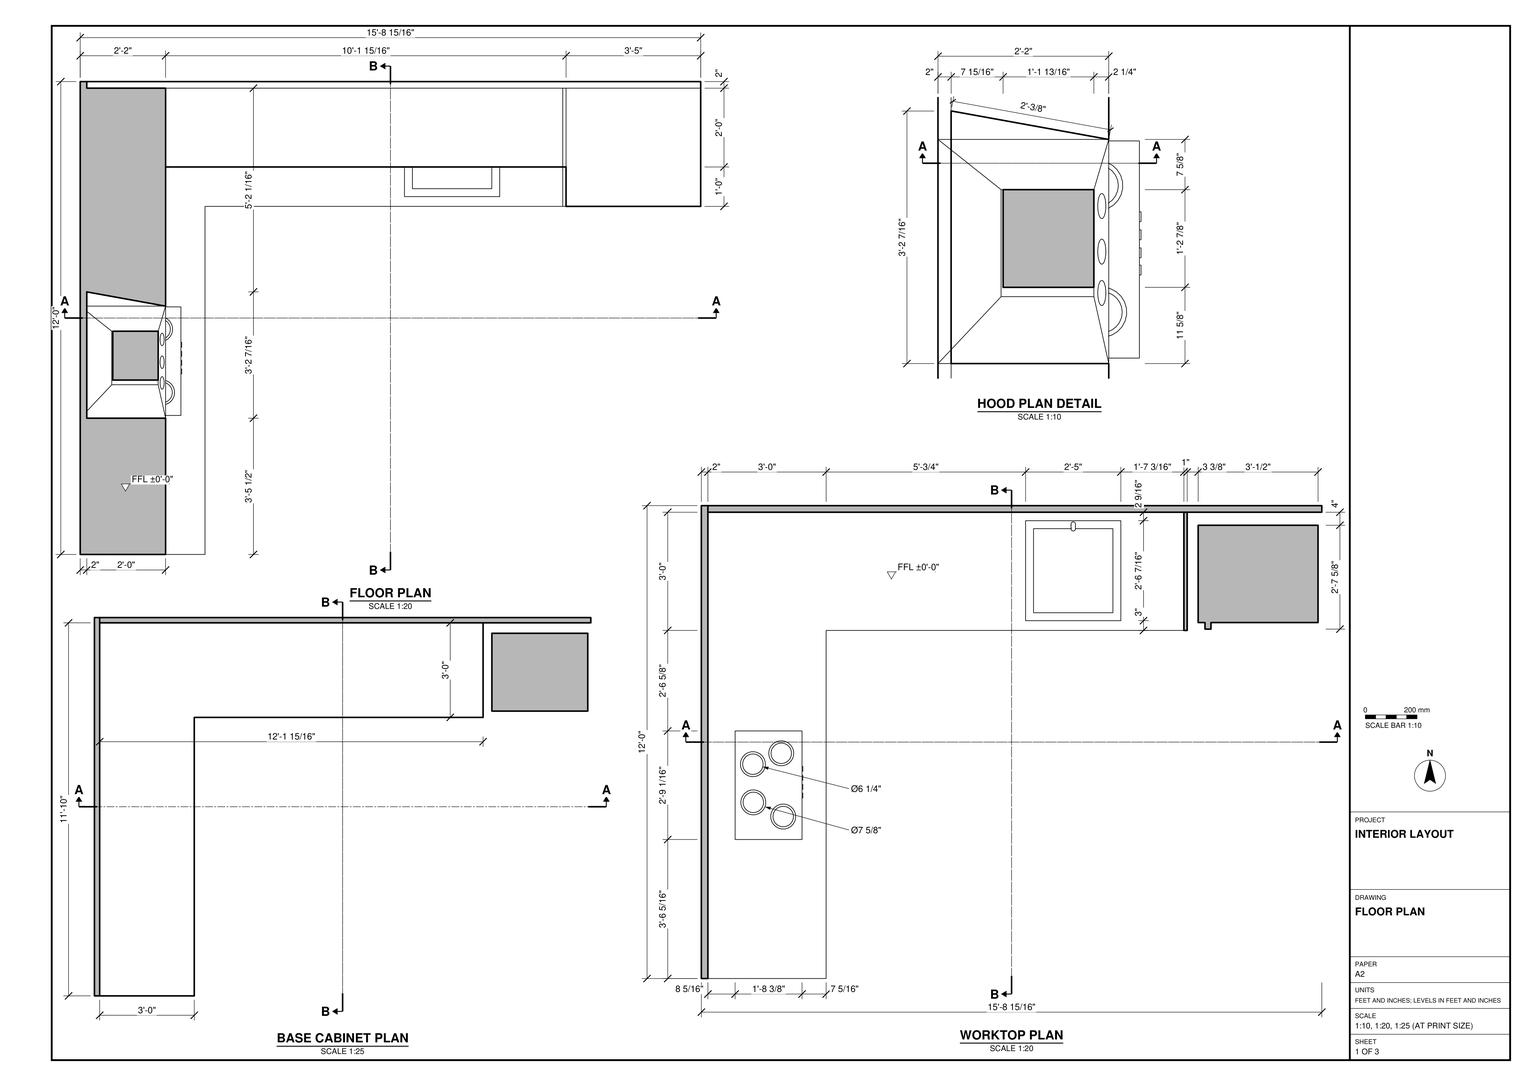
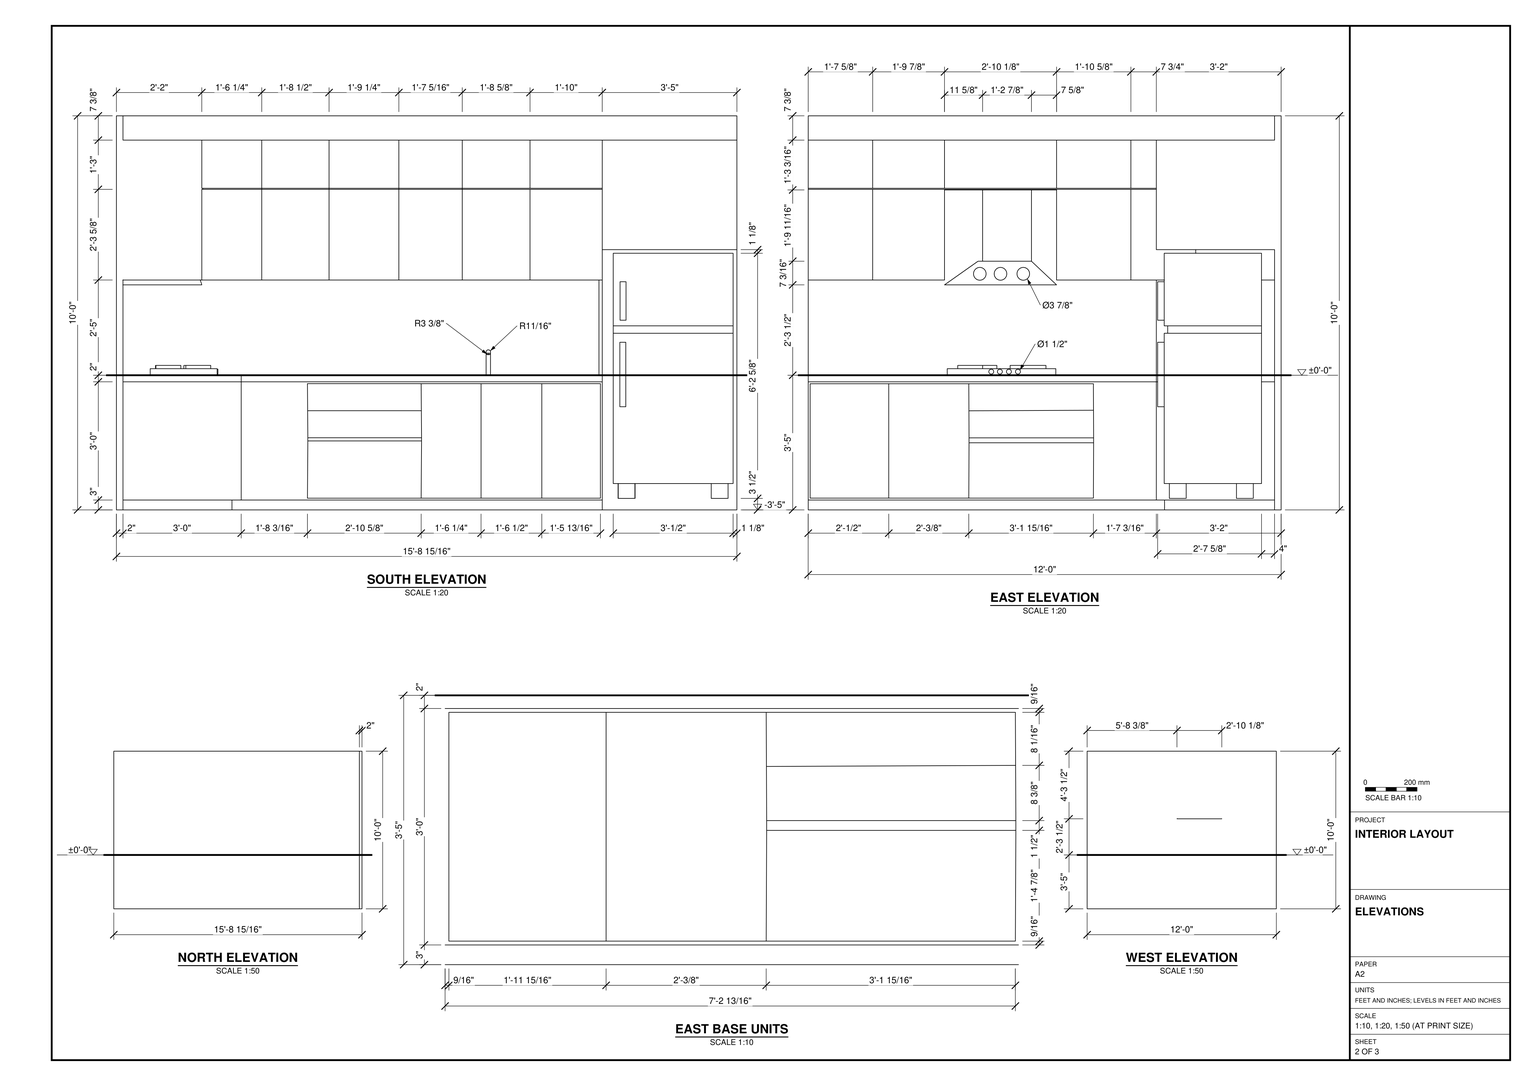
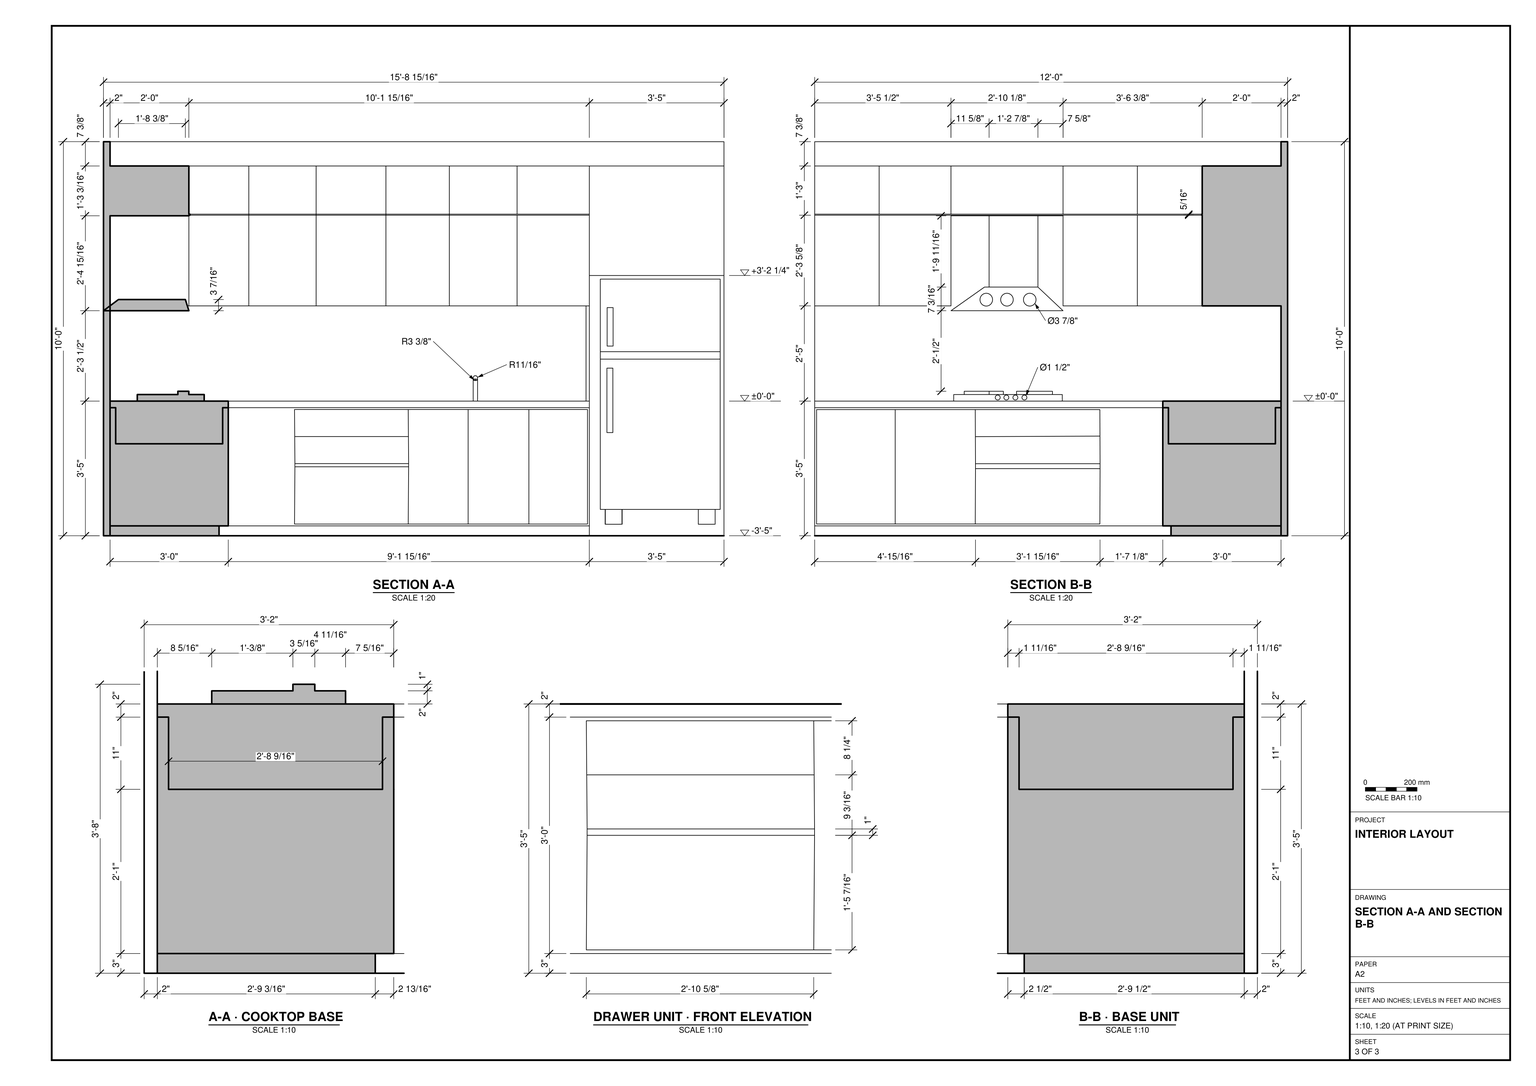
Build the kitchen fit-out in SketchUp from task_files/diagram_01.pdf. Work in feet and inches. Use the single level reference ±0'-0" shown on the sheets. The overall fit-out measures 15'-8 15/16" along the sink wall, 12'-0" along the cooktop wall and 10'-0" in height.

Start with the two perpendicular 2" walls. Use the base cabinet and worktop plans to lay out the L-shaped runs, leaving the refrigerator bay at the far end of the sink wall. Model the worktop, recessed plinths, cupboard fronts and drawer fronts. Use the elevations to distinguish the drawer layout on the sink run from the one on the cooktop run. Fit the sink and tap near the refrigerator, and align the hood above the cooktop on the return. Follow the sections for the depth of the wall cabinets, their clearance above the worktop and the arrangement of fronts around the hood.

Keep each wall, worktop and cabinet unit as a separate group or component, and use components for repeated parts. Appliances, decor and loose items may be any suitable library components. Save one SketchUp model as output_files/l_shaped_kitchen_with_fitted_cabinetry_and_appliances.skp.

# SketchUp Ruby script. Lengths in inches.
U = 1.inch
M = Sketchup.active_model
def pt(a) = Geom::Point3d.new(a.map { |v| v * U })
def face(e, loops, mat)
  f = e.add_face(loops[0].map { |a| pt(a) })
  loops[1..].each { |l| e.add_face(l.map { |a| pt(a) }).erase! }
  f.material = f.back_material = mat if mat
  f
end
# faces: each face lists its corners as indices into pts; further lists are holes
def faces(e, pts, list, mat = nil) = list.each { |f| face(e, (f[0].is_a?(Array) ? f : [f]).map { |l| l.map { |i| pts[i] } }, mat) }
# xy, xz, yz: faces in a plane at the given z, y or x. An outline is a flat list of corners, or four numbers for a rectangle; further outlines are holes
def ring(l) = l.size == 4 ? [[l[0], l[1]], [l[2], l[1]], [l[2], l[3]], [l[0], l[3]]] : l.each_slice(2).to_a
def flat(e, list, mat, &to3) = list.each { |f| face(e, (f[0].is_a?(Array) ? f : [f]).map { |l| ring(l).map { |u, v| to3.(u, v) } }, mat) }
def xy(e, z, list, mat = nil) = flat(e, list, mat) { |x, y| [x, y, z] }
def xz(e, y, list, mat = nil) = flat(e, list, mat) { |x, z| [x, y, z] }
def yz(e, x, list, mat = nil) = flat(e, list, mat) { |y, z| [x, y, z] }
def lines(e, pts, list) = list.each { |a, b| e.add_line(pt(pts[a]), pt(pts[b])) }
# prism: a flat outline (further loops are holes) pulled along v
def prism(e, loops, v, mat = nil)
  f = face(e, loops, mat); d = Geom::Vector3d.new(v.map { |x| x * U })
  f.pushpull(f.normal.samedirection?(d) ? d.length : -d.length)
end
def box(e, o, s, mat = nil) = prism(e, [[o, [o[0] + s[0], o[1], o[2]], [o[0] + s[0], o[1] + s[1], o[2]], [o[0], o[1] + s[1], o[2]]]], [0, 0, s[2]], mat)
def at(x, y, z, deg = 0) = Geom::Transformation.translation(pt([x, y, z])) * Geom::Transformation.rotation(ORIGIN, Z_AXIS, deg.degrees)
def axes(o, x, y, z) = Geom::Transformation.new([*x, 0, *y, 0, *z, 0, *pt(o).to_a, 1])
def part(name) = M.definitions.add(name)
# library, detail: a bought-in or finely detailed component or shape, given as its bounding box
def library(name, o, s) = part(name).tap { |d| box(d.entities, o, s) }
def detail(e, o, s) = box(e.add_group.entities, o, s)
def put(e, d, t, mat = nil) = e.add_instance(d, t).tap { |i| i.material = mat if mat }
def group(e, t, mat = nil) = e.add_group.tap { |g| g.transformation = t; g.material = mat if mat }.entities
root = M.entities
M.materials.add("[0036_BurlyWood]").color = [222, 184, 135]
M.materials.add("[Color M02]").color = [198, 198, 198]
M.materials.add("[Color M06]").color = [86, 86, 86]
M.materials.add("[Color M07]").color = [58, 58, 58]
M.materials.add("[Granite Tile]").color = [155, 148, 143]
M.materials.add("[Marble Carrara Floor Tile]").color = [204, 208, 219]
M.materials.add("[Stone Vein Gray]").color = [166, 165, 165]
c1 = library("Group\#3",[0,0,0],[36.5,31.625,66.0625])
p = [[113.24,138.41,41],[113.24,138.41,47.5],[113.24,138.35,47.66],[113.24,138.26,47.8],[113.24,138.13,47.92],[113.24,137.99,48.01],
  [113.24,137.83,48.0625],[113.24,137.66,48.08],[113.24,137.49,48.0625],[113.24,137.33,48.01],[113.24,137.18,47.92],[113.24,137.0625,47.8],
  [113.24,136.97,47.66],[113.24,136.91,47.5]]
lines(root,p,[[0,1],[1,2],[2,3],[3,4],[4,5],[5,6],[6,7],[7,8],[8,9],[9,10],[10,11],[11,12],
  [12,13]])
detail(root,[10.29,42.33,41],[20.62,33.06,3])
g1 = group(root,at(0,0,0))
xy(g1,0,[[0,0,2,144],[2,0,2,142,147.9375,142,147.9375,108.5,35.1875,108.5,35.1875,0],[2,142,147.9375,144],[147.9375,142,188.9375,144]])
xy(g1,0,[[35.1875,0,35.1875,108.5,147.9375,108.5,147.9375,142,188.9375,142,188.9375,0]],"[Granite Tile]")
xy(g1,3,[[2,0,2,142,147.9375,142,147.9375,108.5,35.1875,108.5,35.1875,0],[35.1875,0,38,108.5],[38,106,147.9375,108.5]])
xy(g1,28,[[3.713,1.713,36.287,1.713,36.287,107.713,146.224,107.713,146.224,140.287,3.713,140.287]])
xy(g1,28.6875,[[101.152,111.388,125.325,136.999]])
xy(g1,39,[[[2,0,2,142,147.9375,142,147.9375,106,38,106,38,0],[3.713,1.713,36.287,1.713,36.287,107.713,146.224,107.713,146.224,140.287,3.713,140.287]]])
xy(g1,41,[[[98.739,108.975,127.739,139.412],[101.152,111.388,125.325,136.999],[113.239,137.739,113.065,137.762,112.904,137.829,112.765,137.935,112.658,138.074,112.591,138.236,112.569,138.409,112.591,138.582,112.658,138.744,112.765,138.883,112.904,138.989,113.065,139.056,113.239,139.079,113.412,139.056,113.573,138.989,113.712,138.883,113.819,138.744,113.886,138.582,113.908,138.409,113.886,138.236,113.819,138.074,113.712,137.935,113.573,137.829,113.412,137.762]],[113.239,137.739,113.065,137.762,112.904,137.829,112.765,137.935,112.658,138.074,112.591,138.236,112.569,138.409,112.591,138.582,112.658,138.744,112.765,138.883,112.904,138.989,113.065,139.056,113.239,139.079,113.412,139.056,113.573,138.989,113.712,138.883,113.819,138.744,113.886,138.582,113.908,138.409,113.886,138.236,113.819,138.074,113.712,137.935,113.573,137.829,113.412,137.762]])
xy(g1,41,[[146.9375,106,147.9375,142]],"[0036_BurlyWood]")
xy(g1,41,[[[2,0,38,0,38,106,146.9375,106,146.9375,142,2,142],[98.739,108.975,127.739,139.412]]],"[Stone Vein Gray]")
xy(g1,70,[[2,0,26,41.497],[26,75.622,2,79.962,2,142,26,142],[146.9375,106,147.9375,118],[26,118,146.9375,142],[146.9375,118,147.9375,142]],"[0036_BurlyWood]")
xy(g1,79.249,[[147.9375,106,188.9375,142]],"[0036_BurlyWood]")
xy(g1,97.4375,[[2,41.497,2,79.962,26,75.622,26,41.497]])
xy(g1,97.613,[[125.9375,117.875,147.9375,118]],"[0036_BurlyWood]")
xy(g1,97.614,[[26,0,26.3125,118],[26.3125,117.875,44.25,118],[44.25,117.875,64.75,118],[64.75,117.875,86,118],[86,117.875,105.3125,118],
  [105.3125,117.875,125.9375,118]],"[0036_BurlyWood]")
xy(g1,97.929,[[26,0,26.3125,118],[26.3125,117.875,44.25,118],[44.25,117.875,64.75,118],[64.75,117.875,86,118],[86,117.875,105.3125,118],
  [105.3125,117.875,147.9375,118]],"[0036_BurlyWood]")
xy(g1,112.601,[[2,0,26,142],[147.9375,106,188.9375,142],[26,118,147.9375,142]],"[0036_BurlyWood]")
xy(g1,120,[[0,0,2,144],[2,142,188.9375,144]])
xz(g1,0,[[2,0,35.1875,3]])
xz(g1,0,[[0,0,2,0,2,70,26,70,26,97.614,26.3125,97.614,26.3125,97.929,26,97.929,26,112.601,2,112.601,2,120,0,120],[2,3,38,39]],"[0036_BurlyWood]")
xz(g1,0,[[2,39,38,41]],"[Stone Vein Gray]")
xz(g1,1.713,[[3.713,28,36.287,39]])
xz(g1,41.497,[[2,70,26,97.4375]],"[0036_BurlyWood]")
xz(g1,106,[[[38,3,147.9375,39],[58.162,3.56,58.287,21,58.287,21.974,58.224,30.207,58.162,38.44,147.378,38.44,147.378,3.56]],[58.162,3.56,92.787,3.56,92.912,21,58.287,21],[92.787,3.56,111.037,3.56,111.037,38.44,92.787,38.44,92.849,30.207,92.912,21.974,92.912,21],[111.037,3.56,129.537,38.44],[129.537,3.56,147.378,38.44],
  [58.287,21,92.912,21.974],[58.287,21.974,92.912,21.974,92.849,30.207,58.224,30.207],[58.224,30.207,92.849,30.207,92.787,38.44,58.162,38.44],[146.9375,41,147.9375,70],[147.9375,79.249,188.9375,112.601]],"[0036_BurlyWood]")
xz(g1,106,[[38,39,147.9375,41]],"[Stone Vein Gray]")
xz(g1,107.713,[[36.287,28,146.224,39]])
xz(g1,108.5,[[35.1875,0,147.9375,3]])
xz(g1,111.388,[[101.152,28.6875,125.325,41]])
xz(g1,117.875,[[125.9375,97.613,147.9375,97.613,147.9375,97.929,105.3125,97.929,105.3125,97.614,125.9375,97.614],[26.3125,97.614,44.25,97.929],[44.25,97.614,64.75,97.929],[64.75,97.614,86,97.929],[86,97.614,105.3125,97.929]],"[0036_BurlyWood]")
xz(g1,118,[[26,97.614,26.3125,97.8],[26,97.8,26.3125,97.929]])
xz(g1,118,[[26,70,44.25,97.614],[44.25,70,64.75,97.614],[64.75,70,86,97.614],[86,70,105.3125,97.614],[105.3125,70,125.9375,97.614],
  [125.9375,70,147.9375,97.613],[26,97.929,44.25,112.601],[44.25,97.929,64.75,112.601],[64.75,97.929,86,112.601],[86,97.929,105.3125,112.601],
  [105.3125,97.929,125.9375,112.601],[125.9375,97.929,147.9375,112.601]],"[0036_BurlyWood]")
xz(g1,136.999,[[101.152,28.6875,125.325,41]])
xz(g1,140.287,[[3.713,28,146.224,39]])
xz(g1,142,[[2,0,147.9375,3],[2,3,147.9375,39],[2,39,147.9375,41],[2,70,26,112.601],[2,112.601,188.9375,120]])
xz(g1,142,[[147.9375,0,188.9375,79.249],[146.9375,41,147.9375,70]],"[0036_BurlyWood]")
xz(g1,142,[[2,41,146.9375,70]],"[Marble Carrara Floor Tile]")
xz(g1,144,[[0,0,2,120],[2,0,188.9375,120]])
yz(g1,0,[[0,0,144,120]])
yz(g1,2,[[0,0,142,3],[142,0,144,120],[0,3,142,39],[0,39,142,41],[0,112.601,142,120]])
yz(g1,2,[[0,41,142,41,142,70,79.962,70,79.962,97.4375,41.497,97.4375,41.497,70,0,70]],"[Marble Carrara Floor Tile]")
yz(g1,3.713,[[1.713,28,140.287,39]])
yz(g1,26,[[118,70,142,112.601],[41.497,97.4375,75.622,97.614]])
yz(g1,26,[[0,70,19.625,97.614],[19.625,70,41.497,97.614],[75.622,70,98.247,97.614],[98.247,70,118,97.614],[0,97.929,19.625,112.601],
  [19.625,97.929,41.497,112.601],[41.497,97.929,75.622,112.601],[75.622,97.929,98.247,112.601],[98.247,97.929,118,112.601]],"[0036_BurlyWood]")
yz(g1,26.3125,[[117.875,97.614,118,97.929]])
yz(g1,26.3125,[[0,97.614,117.875,97.929]],"[0036_BurlyWood]")
yz(g1,35.1875,[[0,0,108.5,3]])
yz(g1,36.287,[[1.713,28,107.713,39]])
yz(g1,38,[[[0,3,106,39],[0.581,3.581,0.581,38.419,86.83,38.419,86.865,30.341,86.901,21.937,86.901,20.438,86.83,3.581]],[0.581,3.581,24.517,38.419],[24.517,3.581,48.892,3.581,48.963,20.438,48.963,21.937,48.928,30.178,48.892,38.419,24.517,38.419],[48.892,3.581,86.83,3.581,86.901,20.438,48.963,20.438],[48.963,20.438,86.901,21.937],
  [48.963,21.937,86.901,21.937,86.865,30.341,48.928,30.178],[48.928,30.178,86.865,30.341,86.83,38.419,48.892,38.419]],"[0036_BurlyWood]")
yz(g1,38,[[0,39,106,41]],"[Stone Vein Gray]")
yz(g1,101.152,[[111.388,28.6875,136.999,41]])
yz(g1,125.325,[[111.388,28.6875,136.999,38.375],[111.388,38.375,136.999,41]])
yz(g1,125.9375,[[117.875,97.613,118,97.614]])
yz(g1,146.224,[[107.713,28,140.287,39]])
yz(g1,146.9375,[[106,41,142,70]],"[0036_BurlyWood]")
yz(g1,147.9375,[[108.5,0,142,3],[106,79.249,106,112.601,118,112.601,118,97.929,117.875,97.929,117.875,97.613,118,97.613,118,79.249]])
yz(g1,147.9375,[[106,3,142,39],[106,41,142,70],[118,70,142,79.249]],"[0036_BurlyWood]")
yz(g1,147.9375,[[106,39,142,41]],"[Stone Vein Gray]")
yz(g1,188.9375,[[142,0,144,0,144,120,142,120,142,112.601,106,112.601,106,79.249,142,79.249]],"[0036_BurlyWood]")
p = [[113.065,137.762,41],[113.239,137.739,41],[113.239,137.739,47.367],[113.239,137.739,47.377],[113.065,137.762,47.381],[113.065,137.762,47.373],
  [113.412,137.762,41],[113.412,137.762,47.373],[113.412,137.762,47.381],[112.765,137.935,41],[112.904,137.829,41],[112.904,137.829,47.394],
  [112.901,137.83,47.394],[112.765,137.935,47.413],[113.573,137.829,41],[113.573,137.829,47.394],[113.712,137.935,41],[113.712,137.935,47.413],
  [113.576,137.83,47.394],[112.658,138.074,41],[112.658,138.074,47.439],[113.819,138.074,41],[113.819,138.074,47.439],[112.591,138.236,41],
  [112.591,138.236,47.468],[113.886,138.236,41],[113.886,138.236,47.468],[112.569,138.409,41],[112.569,138.409,47.5],[113.908,138.409,41],
  [113.908,138.409,47.5],[112.591,138.582,41],[112.591,138.582,47.532],[113.886,138.582,41],[113.886,138.582,47.532],[112.658,138.744,41],
  [112.658,138.744,47.561],[113.819,138.744,41],[113.819,138.744,47.561],[112.765,138.883,41],[112.765,138.883,47.587],[113.712,138.883,41],
  [113.712,138.883,47.587],[112.904,138.989,41],[112.904,138.989,47.606],[113.573,138.989,41],[113.573,138.989,47.606],[113.065,139.056,41],
  [113.065,139.056,47.619],[113.412,139.056,41],[113.412,139.056,47.619],[113.239,139.079,41],[113.239,139.079,47.623],[112.569,136.909,47.5],
  [112.591,137.071,47.439],[112.658,137.222,47.381],[112.765,137.352,47.332],[112.904,137.451,47.294],[113.065,137.514,47.271],[113.239,137.535,47.262],
  [113.412,137.514,47.271],[113.573,137.451,47.294],[113.712,137.352,47.332],[113.819,137.222,47.381],[113.886,137.071,47.439],[113.908,136.909,47.5],
  [113.886,136.747,47.561],[113.819,136.596,47.619],[113.712,136.466,47.668],[113.573,136.366,47.706],[113.412,136.304,47.729],[113.239,136.283,47.738],
  [113.065,136.304,47.729],[112.904,136.366,47.706],[112.765,136.466,47.668],[112.658,136.596,47.619],[112.591,136.747,47.561],[112.658,137.269,47.505],
  [112.765,137.394,47.442],[113.712,137.394,47.442],[113.819,137.269,47.505],[112.904,137.489,47.393],[113.573,137.489,47.393],[113.065,137.549,47.363],
  [113.239,137.569,47.352],[113.412,137.549,47.363],[112.569,136.969,47.659],[112.591,137.125,47.579],[113.886,137.125,47.579],[113.908,136.969,47.659],
  [112.658,137.322,47.586],[112.765,137.429,47.497],[113.712,137.429,47.497],[113.819,137.322,47.586],[112.904,137.512,47.428],[112.765,137.476,47.542],
  [112.904,137.542,47.457],[113.573,137.542,47.457],[113.712,137.476,47.542],[113.573,137.512,47.428],[112.904,137.578,47.479],[113.065,137.606,47.418],
  [113.065,137.583,47.404],[113.065,137.564,47.385],[113.239,137.581,47.371],[113.412,137.564,47.385],[113.412,137.606,47.418],[113.573,137.578,47.479],
  [113.412,137.583,47.404],[112.904,137.659,47.497],[113.065,137.659,47.43],[113.065,137.632,47.427],[112.904,137.617,47.493],[113.239,137.659,47.407],
  [113.239,137.637,47.405],[113.239,137.616,47.397],[113.239,137.597,47.386],[113.412,137.659,47.43],[113.412,137.632,47.427],[113.573,137.659,47.497],
  [113.573,137.617,47.493],[112.904,137.806,47.428],[113.065,137.754,47.385],[113.065,137.735,47.404],[112.904,137.776,47.457],[113.065,137.712,47.418],
  [112.904,137.74,47.479],[113.065,137.686,47.427],[112.904,137.701,47.493],[113.065,137.769,47.363],[113.239,137.749,47.352],[113.239,137.736,47.371],
  [113.239,137.721,47.386],[113.239,137.702,47.397],[113.239,137.681,47.405],[113.412,137.769,47.363],[113.412,137.754,47.385],[113.412,137.735,47.404],
  [113.412,137.712,47.418],[113.412,137.686,47.427],[113.573,137.806,47.428],[113.573,137.776,47.457],[113.573,137.74,47.479],[113.573,137.701,47.493],
  [112.765,137.924,47.442],[112.765,137.888,47.497],[112.765,137.841,47.542],[113.712,137.924,47.442],[113.712,137.888,47.497],[113.712,137.841,47.542],
  [112.658,138.049,47.505],[112.658,137.996,47.586],[113.819,138.049,47.505],[113.819,137.996,47.586],[112.591,138.193,47.579],[113.886,138.193,47.579],
  [112.591,136.814,47.738],[113.886,136.814,47.738],[112.591,137.197,47.689],[113.886,137.197,47.689],[112.658,137.391,47.652],[113.819,137.391,47.652],
  [112.658,137.473,47.702],[112.765,137.532,47.576],[113.712,137.532,47.576],[113.819,137.473,47.702],[112.765,137.594,47.597],[113.712,137.594,47.597],
  [112.765,137.659,47.604],[113.712,137.659,47.604],[112.765,137.786,47.576],[112.765,137.724,47.597],[113.712,137.786,47.576],[113.712,137.724,47.597],
  [112.658,137.927,47.652],[112.658,137.845,47.702],[113.819,137.927,47.652],[113.819,137.845,47.702],[112.591,138.121,47.689],[113.886,138.121,47.689],
  [112.569,138.349,47.659],[113.908,138.349,47.659],[112.591,138.504,47.738],[113.886,138.504,47.738],[112.658,138.649,47.812],[113.819,138.649,47.812],
  [112.765,136.545,47.876],[112.658,136.669,47.812],[113.819,136.669,47.812],[113.712,136.545,47.876],[112.569,137.0625,47.801],[113.908,137.0625,47.801],
  [112.591,137.291,47.781],[113.886,137.291,47.781],[112.658,137.564,47.733],[113.819,137.564,47.733],[112.658,137.659,47.744],[113.819,137.659,47.744],
  [112.658,137.754,47.733],[113.819,137.754,47.733],[112.591,138.026,47.781],[113.886,138.026,47.781],[112.569,138.255,47.801],[113.908,138.255,47.801],
  [112.765,138.773,47.876],[113.712,138.773,47.876],[112.904,138.869,47.924],[113.573,138.869,47.924],[113.065,138.928,47.955],[113.239,138.949,47.965],
  [113.412,138.928,47.955],[113.065,136.389,47.955],[112.904,136.449,47.924],[113.239,136.369,47.965],[113.412,136.389,47.955],[113.573,136.449,47.924],
  [112.658,136.803,48.016],[112.591,136.928,47.912],[113.886,136.928,47.912],[113.819,136.803,48.016],[112.569,137.185,47.919],[113.908,137.185,47.919],
  [112.591,137.404,47.85],[113.886,137.404,47.85],[112.591,137.528,47.892],[113.886,137.528,47.892],[112.591,137.659,47.907],[113.886,137.659,47.907],
  [112.591,137.79,47.892],[113.886,137.79,47.892],[112.591,137.914,47.85],[113.886,137.914,47.85],[112.569,138.133,47.919],[113.908,138.133,47.919],
  [112.591,138.39,47.912],[113.886,138.39,47.912],[112.658,138.515,48.016],[113.819,138.515,48.016],[112.765,136.696,48.105],[113.712,136.696,48.105],
  [112.591,137.078,48.057],[113.886,137.078,48.057],[112.569,137.329,48.007],[113.908,137.329,48.007],[112.569,137.49,48.0625],[113.908,137.49,48.0625],
  [112.569,137.988,48.007],[112.569,137.828,48.0625],[113.908,137.988,48.007],[113.908,137.828,48.0625],[112.591,138.24,48.057],[113.886,138.24,48.057],
  [112.765,138.622,48.105],[113.712,138.622,48.105],[112.904,136.613,48.173],[113.065,136.561,48.216],[113.573,136.613,48.173],[113.412,136.561,48.216],
  [112.658,136.978,48.185],[113.819,136.978,48.185],[112.591,137.255,48.165],[113.886,137.255,48.165],[112.569,137.659,48.081],[113.908,137.659,48.081],
  [112.591,138.0625,48.165],[113.886,138.0625,48.165],[112.658,138.34,48.185],[113.819,138.34,48.185],[112.904,138.705,48.173],[113.573,138.705,48.173],
  [113.065,138.757,48.216],[113.412,138.757,48.216],[113.239,136.544,48.231],[112.765,136.893,48.296],[113.712,136.893,48.296],[112.591,137.452,48.233],
  [113.886,137.452,48.233],[112.591,137.866,48.233],[113.886,137.866,48.233],[112.765,138.425,48.296],[113.712,138.425,48.296],[113.239,138.774,48.231],
  [112.904,136.827,48.38],[113.573,136.827,48.38],[112.658,137.186,48.3125],[113.819,137.186,48.3125],[112.591,137.659,48.255],[113.886,137.659,48.255],
  [112.658,138.132,48.3125],[113.819,138.132,48.3125],[112.904,138.491,48.38],[113.573,138.491,48.38],[113.239,136.772,48.452],[113.065,136.786,48.433],
  [113.412,136.786,48.433],[112.765,137.127,48.439],[113.712,137.127,48.439],[112.658,137.417,48.391],[113.819,137.417,48.391],[112.658,137.659,48.418],
  [113.819,137.659,48.418],[112.658,137.901,48.391],[113.819,137.901,48.391],[112.765,138.191,48.439],[113.712,138.191,48.439],[113.065,138.532,48.433],
  [113.239,138.546,48.452],[113.412,138.532,48.433],[112.904,137.081,48.536],[113.573,137.081,48.536],[112.765,137.386,48.527],[113.712,137.386,48.527],
  [112.765,137.932,48.527],[113.712,137.932,48.527],[112.904,138.237,48.536],[113.573,138.237,48.536],[113.065,137.053,48.597],[113.239,137.043,48.617],
  [113.412,137.053,48.597],[112.904,137.363,48.632],[113.573,137.363,48.632],[112.765,137.659,48.558],[113.712,137.659,48.558],[112.904,137.955,48.632],
  [113.573,137.955,48.632],[113.065,138.265,48.597],[113.412,138.265,48.597],[113.239,138.275,48.617],[113.065,137.348,48.698],[113.412,137.348,48.698],
  [112.904,137.659,48.665],[113.573,137.659,48.665],[113.065,137.97,48.698],[113.412,137.97,48.698],[113.239,137.343,48.72],[113.065,137.659,48.732],
  [113.412,137.659,48.732],[113.239,137.975,48.72],[113.239,137.659,48.755],[2,79.962,70],[26,75.622,70],[26,75.622,97.4375],
  [2,79.962,97.4375],[146.224,140.287,39],[146.224,140.287,41],[3.713,140.287,39],[3.713,140.287,41],[36.287,1.713,39],
  [36.287,1.713,41],[36.287,107.713,39],[36.287,107.713,41],[146.224,107.713,39],[146.224,107.713,41],[3.713,1.713,39],
  [3.713,1.713,41]]
faces(g1,p,[[0,1,2,3,4,5],[1,6,7,8,3,2],[9,10,11,12,13],[10,0,5,4,11],[6,14,15,8,7],[14,16,17,18,15],[19,9,13,20],[16,21,22,17],
  [23,19,20,24],[21,25,26,22],[27,23,24,28],[25,29,30,26],[31,27,28,32],[29,33,34,30],[35,31,32,36],[33,37,38,34],
  [39,35,36,40],[37,41,42,38],[43,39,40,44],[41,45,46,42],[47,43,44,48],[45,49,50,46],[51,47,48,52],[49,51,52,50],
  [77,78,56,55],[79,80,63,62],[78,81,57,56],[82,79,62,61],[81,83,58,57],[83,84,59,58],[84,85,60,59],[85,82,61,60],
  [86,87,54,53],[88,89,65,64],[87,77,55,54],[80,88,64,63],[90,91,78,77],[92,93,80,79],[91,94,81,78],[95,96,94,91],
  [97,98,92,99],[99,92,79,82],[100,101,102,96],[96,102,103,94],[94,103,83,81],[103,104,84,83],[104,105,85,84],[106,107,97,108],
  [108,97,99,105],[105,99,82,85],[109,110,111,112],[112,111,101,100],[110,113,114,111],[111,114,115,101],[101,115,116,102],[102,116,104,103],
  [113,117,118,114],[114,118,106,115],[115,106,108,116],[116,108,105,104],[117,119,120,118],[118,120,107,106],[121,122,123,124],[124,123,125,126],
  [126,125,127,128],[128,127,110,109],[129,130,2,131,122,5],[122,131,132,123],[123,132,133,125],[125,133,134,127],[127,134,113,110],[130,135,7,136,131,2],
  [131,136,137,132],[132,137,138,133],[133,138,139,134],[134,139,117,113],[136,140,141,137],[137,141,142,138],[138,142,143,139],[139,143,119,117],
  [144,12,11,121,145],[144,13,12],[145,121,124,146],[11,129,5,122,121],[135,15,140,136,7],[15,18,147,148,140],[17,147,18],[140,148,149,141],
  [150,144,145,151],[20,13,144,150],[147,152,153,148],[17,22,152,147],[24,20,150,154],[22,26,155,152],[156,86,53,76],[89,157,66,65],
  [158,90,77,87],[93,159,88,80],[160,95,91,90],[98,161,93,92],[162,163,95,160],[164,165,161,98],[166,112,100,163],[163,100,96,95],
  [120,167,164,107],[107,164,98,97],[168,109,112,166],[119,169,167,120],[146,124,126,170],[170,126,128,171],[171,128,109,168],[141,149,172,142],
  [142,172,173,143],[143,173,169,119],[151,145,146,174],[174,146,170,175],[148,153,176,149],[149,176,177,172],[154,150,151,178],[152,155,179,153],
  [28,24,154,180],[26,30,181,155],[32,28,180,182],[30,34,183,181],[36,32,182,184],[34,38,185,183],[186,187,75,74],[188,189,68,67],
  [187,156,76,75],[157,188,67,66],[190,158,87,86],[159,191,89,88],[192,160,90,158],[161,193,159,93],[194,166,163,162],[167,195,165,164],
  [196,168,166,194],[169,197,195,167],[175,170,171,198],[198,171,168,196],[172,177,199,173],[173,199,197,169],[178,151,174,200],[153,179,201,176],
  [180,154,178,202],[155,181,203,179],[40,36,184,204],[38,42,205,185],[44,40,204,206],[42,46,207,205],[48,44,206,208],[52,48,208,209],
  [50,52,209,210],[46,50,210,207],[211,212,73,72],[213,211,72,71],[214,213,71,70],[215,214,70,69],[212,186,74,73],[189,215,69,68],
  [216,217,156,187],[218,219,188,157],[217,190,86,156],[191,218,157,89],[220,192,158,190],[193,221,191,159],[222,162,160,192],[165,223,193,161],
  [224,194,162,222],[195,225,223,165],[226,196,194,224],[197,227,225,195],[228,198,196,226],[199,229,227,197],[200,174,175,230],[230,175,198,228],
  [176,201,231,177],[177,231,229,199],[202,178,200,232],[179,203,233,201],[182,180,202,234],[181,183,235,203],[184,182,234,236],[183,185,237,235],
  [238,216,187,186],[219,239,189,188],[240,220,190,217],[221,241,218,191],[242,222,192,220],[223,243,221,193],[244,224,222,242],[225,245,243,223],
  [246,230,228,247],[231,248,249,229],[232,200,230,246],[201,233,248,231],[234,202,232,250],[203,235,251,233],[204,184,236,252],[185,205,253,237],
  [254,238,186,212],[255,254,212,211],[256,257,214,215],[239,256,215,189],[258,240,217,216],[241,259,219,218],[260,242,220,240],[243,261,241,221],
  [262,226,224,244],[227,263,245,225],[247,228,226,262],[229,249,263,227],[250,232,246,264],[233,251,265,248],[236,234,250,266],[235,237,267,251],
  [206,204,252,268],[205,207,269,253],[208,206,268,270],[207,210,271,269],[272,255,211,213],[257,272,213,214],[273,258,216,238],[259,274,239,219],
  [275,244,242,260],[245,276,261,243],[264,246,247,277],[248,265,278,249],[252,236,266,279],[237,253,280,267],[209,208,270,281],[210,209,281,271],
  [282,273,238,254],[274,283,256,239],[284,260,240,258],[261,285,259,241],[286,262,244,275],[263,287,276,245],[277,247,262,286],[249,278,287,263],
  [266,250,264,288],[251,267,289,265],[268,252,279,290],[253,269,291,280],[292,293,255,272],[294,292,272,257],[293,282,254,255],[283,294,257,256],
  [295,284,258,273],[285,296,274,259],[297,275,260,284],[276,298,285,261],[299,286,275,297],[287,300,298,276],[301,277,286,299],[278,302,300,287],
  [288,264,277,301],[265,289,302,278],[279,266,288,303],[267,280,304,289],[270,268,290,305],[281,270,305,306],[271,281,306,307],[269,271,307,291],
  [308,295,273,282],[296,309,283,274],[310,297,284,295],[298,311,296,285],[303,288,301,312],[289,304,313,302],[290,279,303,314],[280,291,315,304],
  [316,308,282,293],[317,316,293,292],[318,317,292,294],[309,318,294,283],[319,310,295,308],[311,320,309,296],[321,299,297,310],[300,322,311,298],
  [312,301,299,321],[302,313,322,300],[314,303,312,323],[304,315,324,313],[305,290,314,325],[291,307,326,315],[306,305,325,327],[307,306,327,326],
  [328,319,308,316],[320,329,318,309],[330,321,310,319],[322,331,320,311],[323,312,321,330],[313,324,331,322],[325,314,323,332],[315,326,333,324],
  [334,328,316,317],[329,334,317,318],[335,330,319,328],[331,336,329,320],[332,323,330,335],[324,333,336,331],[327,325,332,337],[326,327,337,333],
  [338,335,328,334],[336,338,334,329],[337,332,335,338],[333,337,338,336]],"[Color M06]")
faces(g1,p,[[53,54,55,56,57,58,59,60,61,62,63,64,65,66,67,68,69,70,71,72,73,74,75,76]])
faces(g1,p,[[339,340,341,342]],"[0036_BurlyWood]")
lines(g1,p,[[343,344],[345,346],[347,348],[349,350],[351,352],[353,354]])
g2 = group(g1,at(9.91,53.1,75.72))
box(g2,[0,0,0],[13.82,14.875,21.72],"[Color M07]")
g3 = group(g1,at(0,41.5,68.52))
xy(g3,0,[[[0,0,26,34.125],[1.92,1.52,24.08,32.61]],[1.92,1.52,24.08,32.61]],"[Color M07]")
xy(g3,7.2,[[9.61,10.1875,23.74,26.48]],"[Color M07]")
p = [[0,0,0],[9.61,10.1875,7.2],[9.61,26.48,7.2],[0,34.125,0],[26,0,0],[23.74,10.1875,7.2],
  [26,34.125,0],[23.74,26.48,7.2],[24.33,10.94,5.32],[24.36,11.42,5.21],[24.4375,11.87,4.97],[24.55,12.23,4.62],
  [24.68,12.5,4.18],[24.84,12.64,3.69],[25,12.66,3.18],[25.16,12.55,2.68],[25.3,12.3125,2.23],[25.42,11.97,1.86],
  [25.5,11.54,1.59],[25.55,11.0625,1.44],[25.55,10.5625,1.42],[25.52,10.07,1.54],[25.44,9.63,1.78],[25.33,9.26,2.13],
  [25.19,9,2.5625],[25.04,8.85,3.05],[24.88,8.84,3.5625],[24.72,8.95,4.06],[24.58,9.1875,4.51],[24.46,9.53,4.89],
  [24.38,9.95,5.16],[24.33,10.43,5.3],[24.84,18.94,3.69],[25,18.96,3.18],[25.16,18.85,2.68],[25.3,18.61,2.23],
  [25.42,18.27,1.86],[25.5,17.84,1.59],[25.55,17.36,1.44],[25.55,16.86,1.42],[25.52,16.37,1.54],[25.44,15.93,1.78],
  [25.33,15.5625,2.13],[25.19,15.3,2.5625],[25.04,15.15,3.05],[24.88,15.13,3.5625],[24.72,15.25,4.06],[24.58,15.48,4.51],
  [24.46,15.83,4.89],[24.38,16.25,5.16],[24.33,16.73,5.3],[24.33,17.23,5.32],[24.36,17.72,5.21],[24.4375,18.17,4.97],
  [24.55,18.53,4.62],[24.68,18.8,4.18],[24.84,25.88,3.69],[25,25.9,3.18],[25.16,25.79,2.68],[25.3,25.55,2.23],
  [25.42,25.21,1.86],[25.5,24.78,1.59],[25.55,24.3,1.44],[25.55,23.8,1.42],[25.52,23.3125,1.54],[25.44,22.87,1.78],
  [25.33,22.5,2.13],[25.19,22.24,2.5625],[25.04,22.09,3.05],[24.88,22.07,3.5625],[24.72,22.1875,4.06],[24.58,22.42,4.51],
  [24.46,22.77,4.89],[24.38,23.19,5.16],[24.33,23.67,5.3],[24.33,24.17,5.32],[24.36,24.66,5.21],[24.4375,25.1,4.97],
  [24.55,25.47,4.62],[24.68,25.74,4.18]]
faces(g3,p,[[0,1,2,3],[0,4,5,1],[[4,6,7,5],[8,9,10,11,12,13,14,15,16,17,18,19,20,21,22,23,24,25,26,27,28,29,30,31],[32,33,34,35,36,37,38,39,40,41,42,43,44,45,46,47,48,49,50,51,52,53,54,55],[56,57,58,59,60,61,62,63,64,65,66,67,68,69,70,71,72,73,74,75,76,77,78,79]],[3,2,7,6]],"[Color M07]")
faces(g3,p,[[9,8,31,30,29,28,27,26,25,24,23,22,21,20,19,18,17,16,15,14,13,12,11,10],[52,51,50,49,48,47,46,45,44,43,42,41,40,39,38,37,36,35,34,33,32,55,54,53],[76,75,74,73,72,71,70,69,68,67,66,65,64,63,62,61,60,59,58,57,56,79,78,77]],"[Color M02]")
put(g1,c1,axes([151.28,106.4,3.5],[1,0,0],[0,1,0],[0,0,1.13]))
